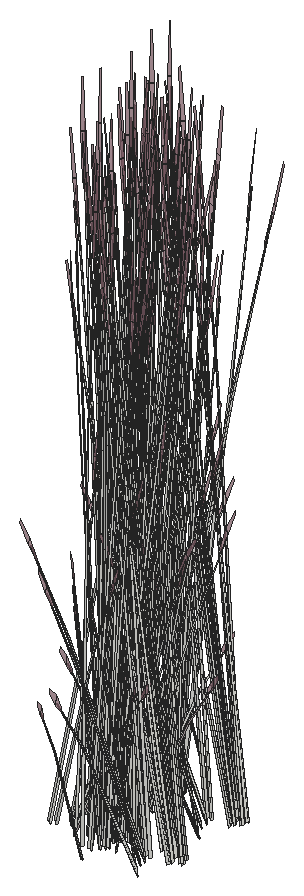
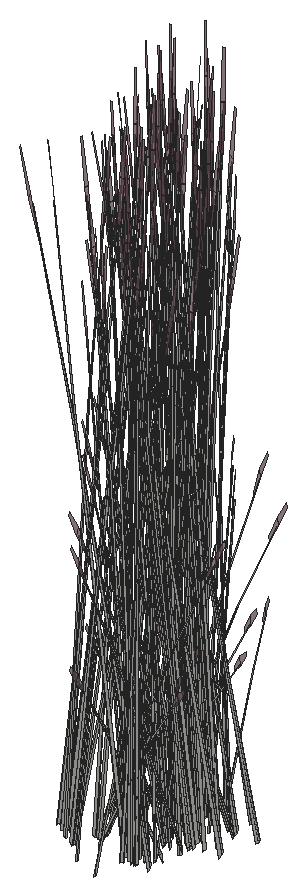
# SketchUp Ruby script. Lengths in inches.
U = 1.inch
M = Sketchup.active_model
def pt(a) = Geom::Point3d.new(a.map { |v| v * U })
def face(e, loops, mat)
  f = e.add_face(loops[0].map { |a| pt(a) })
  loops[1..].each { |l| e.add_face(l.map { |a| pt(a) }).erase! }
  f.material = f.back_material = mat if mat
  f
end
# faces: each face lists its corners as indices into pts; further lists are holes
def faces(e, pts, list, mat = nil) = list.each { |f| face(e, (f[0].is_a?(Array) ? f : [f]).map { |l| l.map { |i| pts[i] } }, mat) }
# xy, xz, yz: faces in a plane at the given z, y or x. An outline is a flat list of corners, or four numbers for a rectangle; further outlines are holes
def ring(l) = l.size == 4 ? [[l[0], l[1]], [l[2], l[1]], [l[2], l[3]], [l[0], l[3]]] : l.each_slice(2).to_a
def flat(e, list, mat, &to3) = list.each { |f| face(e, (f[0].is_a?(Array) ? f : [f]).map { |l| ring(l).map { |u, v| to3.(u, v) } }, mat) }
def xy(e, z, list, mat = nil) = flat(e, list, mat) { |x, y| [x, y, z] }
def xz(e, y, list, mat = nil) = flat(e, list, mat) { |x, z| [x, y, z] }
def yz(e, x, list, mat = nil) = flat(e, list, mat) { |y, z| [x, y, z] }
def lines(e, pts, list) = list.each { |a, b| e.add_line(pt(pts[a]), pt(pts[b])) }
# prism: a flat outline (further loops are holes) pulled along v
def prism(e, loops, v, mat = nil)
  f = face(e, loops, mat); d = Geom::Vector3d.new(v.map { |x| x * U })
  f.pushpull(f.normal.samedirection?(d) ? d.length : -d.length)
end
def box(e, o, s, mat = nil) = prism(e, [[o, [o[0] + s[0], o[1], o[2]], [o[0] + s[0], o[1] + s[1], o[2]], [o[0], o[1] + s[1], o[2]]]], [0, 0, s[2]], mat)
def at(x, y, z, deg = 0) = Geom::Transformation.translation(pt([x, y, z])) * Geom::Transformation.rotation(ORIGIN, Z_AXIS, deg.degrees)
def axes(o, x, y, z) = Geom::Transformation.new([*x, 0, *y, 0, *z, 0, *pt(o).to_a, 1])
def part(name) = M.definitions.add(name)
# library, detail: a bought-in or finely detailed component or shape, given as its bounding box
def library(name, o, s) = part(name).tap { |d| box(d.entities, o, s) }
def detail(e, o, s) = box(e.add_group.entities, o, s)
def put(e, d, t, mat = nil) = e.add_instance(d, t).tap { |i| i.material = mat if mat }
def group(e, t, mat = nil) = e.add_group.tap { |g| g.transformation = t; g.material = mat if mat }.entities
root = M.entities
M.materials.add("LightPink_Translucent").color = [144, 107, 117]
M.materials["LightPink_Translucent"].alpha = 0.75
c1 = part("blade")
p = [[2.15,0.21,22],[0,0.17,0],[0.09,0.45,0],[2.18,0.31,22],[2.29,0.31,22],[0.38,0.45,0],
  [2.48,0.24,33],[2.49,0.24,33],[2.48,0.22,33]]
faces(c1.entities,p,[[0,1,2,3],[4,5,2,3],[6,3,4,7],[8,0,3,6]])
c2 = part("seeds")
p = [[0.3,-0.1,1.38],[-0.01,-0.03,1.59],[-0.01,-0.03,0.03],[0.14,-0.07,-0.07],[0.29,-0.03,3],[0.15,0.01,3.11]]
faces(c2.entities,p,[[0,1,2,3],[1,0,4,5]],"LightPink_Translucent")
c3 = part("blade with seeds")
put(c3.entities,c1,at(0,0,0))
put(c3.entities,c2,axes([2.4,0.25,30.99],[1.5799,-0.05474,1.17369],[-0.12525,1.92788,0.29478],[-0.07173,-0.02425,1.56792]))
put(root,c3,axes([333.875,17.01,50.09],[0.63817,0.08233,0.40429],[-0.12987,0.46497,0.15865],[-0.09326,-0.0449,1.40366]))
put(root,c3,axes([332.37,20.08,50.3125],[0.47043,-0.11396,0.12794],[0.16474,0.32541,-0.36534],[0,0.07162,1.11991]))
put(root,c3,axes([329.59,16.35,49.82],[0.52523,0.06406,-0.55095],[-0.11084,0.39517,-0.1446],[0.15674,0.04788,1.21613]))
put(root,c3,axes([331.83,16.59,50],[-0.31304,-0.24986,-0.05733],[0.34284,-0.22894,-0.25992],[0.09714,-0.01612,0.85731]))
put(root,c3,axes([333.71,16.93,50.4],[-0.24498,0.3521,0.39531],[-0.50902,-0.16945,-0.19025],[0,-0.08116,1.26923]))
put(root,c3,axes([332.21,20.11,50.36],[0.56863,0.18645,-0.25709],[-0.2738,0.39352,-0.44182],[0.01787,0.09662,1.41118]))
put(root,c3,axes([331,18.77,49.79],[0.47106,0.09668,-0.27372],[-0.11861,0.34048,0.27372],[0.09497,-0.03926,1.22797]))
put(root,c3,axes([332.3125,18.36,50.29],[-0.14352,0.07909,1.26356],[-0.42983,-0.13843,-0.27174],[0.07968,-0.17216,0.54024]))
put(root,c3,axes([333.53,17.75,50.1875],[0.54257,-0.10371,0.15589],[0.13397,0.38597,0.31002],[-0.04839,-0.05624,1.41735]))
put(root,c3,axes([334.36,24.57,50.03],[-0.46965,-0.33633,-0.05417],[0.46994,-0.33653,0],[-0.0164,-0.01174,1.55135]))
put(root,c3,axes([334.23,17.82,49.94],[-0.50902,-0.17543,0],[0.24498,-0.36452,0],[0,0,1.43768]))
put(root,c3,axes([333.45,20.2,50.19],[0,-0.39075,0.43871],[0.56491,0,0],[0,0.089,1.3917]))
put(root,c3,axes([333.6875,20.56,49.78],[0,0.39075,-0.43871],[-0.56491,0,0],[0,0.089,1.3917]))
put(root,c3,axes([335.41,18.25,50.1],[0.31568,0.39156,0],[-0.52815,0.21836,-0.456],[-0.12029,0.04973,1.44655]))
put(root,c3,axes([330.89,18.61,49.78],[0.47255,-0.19538,-0.43871],[0.28245,0.35034,0],[0.10763,-0.0445,1.3917]))
put(root,c3,axes([337.74,15.88,50.29],[0.09858,0.10879,1.26356],[-0.22716,0.29571,-0.27174],[-0.23325,-0.07068,0.54024]))
put(root,c3,axes([337.74,22.16,50.29],[0.09858,0.10879,1.26356],[-0.22716,0.29571,-0.27174],[-0.23325,-0.07068,0.54024]))
put(root,c3,axes([333.7,22.125,49.32],[-0.08469,0.01408,1.55816],[-0.46834,-0.15847,-0.23804],[0.00786,-0.13218,0.26541]))
put(root,c3,axes([331.84,19.58,50.3125],[0.09741,-0.34873,0.12794],[0.4759,0.06053,-0.36534],[0.08661,0.03581,1.11991]))
put(root,c3,axes([333.42,24.18,50.09],[0.21952,0.43694,0.40429],[-0.62724,0.15194,0.15865],[0.00767,-0.08029,1.40366]))
put(root,c3,axes([333.32,24.125,49.95],[0.24498,-0.3521,-0.39531],[0.50902,0.16945,0.19025],[0,-0.08116,1.26923]))
put(root,c3,axes([335.15,17.77,50.1875],[0.14586,-0.38834,0.15589],[0.53375,0.1099,0.31002],[-0.0922,0.00189,1.41735]))
put(root,c3,axes([334.9,17.26,50.3125],[0.37303,0.23477,0.12794],[-0.31115,0.26487,-0.36534],[-0.08661,0.03581,1.11991]))
put(root,c3,axes([332.51,18.98,50.19],[-0.47255,-0.19538,0.43871],[0.28245,-0.35034,0],[0.10763,0.0445,1.3917]))
put(root,c3,axes([334.77,16.97,50.03],[-0.46965,-0.33633,-0.05417],[0.46994,-0.33653,0],[-0.0164,-0.01174,1.55135]))
put(root,c3,axes([334.89,17.09,50.4],[0.54829,-0.02412,0.39531],[0.04958,0.40041,-0.19025],[-0.09816,0.04058,1.26923]))
put(root,c3,axes([332.1,21.02,49.93],[0.53009,-0.13258,-0.16963],[0.18627,0.38191,0.00007],[0.05851,-0.01465,1.53656]))
put(root,c3,axes([335.02,18.01,50.06],[0.63212,0.12701,0.27176],[-0.15814,0.45398,-0.32244],[-0.10462,0.05682,1.45692]))
put(root,c3,axes([334.1,14.53,49.32],[-0.08469,0.01408,1.55816],[-0.46834,-0.15847,-0.23804],[0.00786,-0.13218,0.26541]))
put(root,c3,axes([337.39,16.61,49.32],[0.0128,0.06158,1.55816],[-0.25814,0.3216,-0.23804],[-0.18336,-0.01621,0.26541]))
put(root,c3,axes([337.39,22.89,49.32],[0.0128,0.06158,1.55816],[-0.25814,0.3216,-0.23804],[-0.18336,-0.01621,0.26541]))
put(root,c3,axes([335.3,17.98,50.19],[0.47255,-0.19538,0.43871],[0.28245,0.35034,0],[-0.10763,0.0445,1.3917]))
put(root,c3,axes([333.82,16.58,50.09],[0.21952,0.43694,0.40429],[-0.62724,0.15194,0.15865],[0.00767,-0.08029,1.40366]))
put(root,c3,axes([333.72,16.53,49.95],[0.24498,-0.3521,-0.39531],[0.50902,0.16945,0.19025],[0,-0.08116,1.26923]))
put(root,c3,axes([334.35,17.66,49.95],[-0.16474,-0.33688,0],[0.47043,-0.11798,0],[0,0,1.36402]))
put(root,c3,axes([333.75,18.375,49.32],[0.08172,-0.02126,1.55816],[0.49154,0.11703,-0.23804],[0.01437,0.1319,0.26541]))
put(root,c3,axes([332.11,19.88,49.95],[0.30332,0.32798,-0.39531],[-0.45944,0.23096,0.19025],[0.09816,0.04058,1.26923]))
put(root,c3,axes([334.21,24.22,49.95],[0,-0.45213,0],[0.63136,0,0],[0,0,1.58567]))
put(root,c3,axes([333.62,24.3,50.15],[0.56891,0.18939,0.21263],[-0.2738,0.39352,0.44182],[0,-0.09071,1.41855]))
put(root,c3,axes([333.44,24.04,50.4],[-0.54829,0.02412,0.39531],[-0.04958,-0.40041,-0.19025],[0.09816,-0.04058,1.26923]))
put(root,c3,axes([331.96,21.25,50.29],[0.00891,-0.12953,1.26356],[0.4258,-0.14469,-0.27174],[0.13144,0.15503,0.54024]))
put(root,c3,axes([331.45,19.41,49.82],[0.34009,-0.2937,-0.55095],[0.42248,0.26632,-0.1446],[0.13628,-0.07327,1.21613]))
put(root,c3,axes([333.18,23.35,50.1875],[-0.14586,0.38834,0.15589],[-0.53375,-0.1099,0.31002],[0.0922,-0.00189,1.41735]))
put(root,c3,axes([335.01,17,49.95],[-0.24498,0.3521,-0.39531],[-0.50902,-0.16945,0.19025],[0,0.08116,1.26923]))
put(root,c3,axes([330.9,15.89,50.29],[-0.18038,-0.01157,1.26356],[-0.18479,-0.31048,-0.27174],[0.22159,-0.08783,0.54024]))
put(root,c3,axes([337.25,18.34,49.32],[0.06773,0.03904,1.55816],[0.11484,0.36171,-0.23804],[-0.15011,0.07713,0.26541]))
put(root,c3,axes([335.98,16.78,50.1875],[-0.39671,-0.28463,0.15589],[0.39978,-0.27607,0.31002],[-0.04381,0.05813,1.41735]))
put(root,c3,axes([332.94,19.15,49.79],[0.11861,0.34048,-0.27372],[-0.47106,0.09668,0.27372],[0.09497,0.03926,1.22797]))
put(root,c3,axes([334.61,16.62,49.95],[0,-0.45213,0],[0.63136,0,0],[0,0,1.58567]))
put(root,c3,axes([333.83,20.26,50.1],[0.63136,0,0],[0,0.43672,-0.456],[0,0.09947,1.44655]))
put(root,c3,axes([332.92,22.87,50.1],[-0.31568,-0.39156,0],[0.52815,-0.21836,-0.456],[0.12029,-0.04973,1.44655]))
put(root,c3,axes([334.02,16.7,50.15],[0.56891,0.18939,0.21263],[-0.2738,0.39352,0.44182],[0,-0.09071,1.41855]))
put(root,c3,axes([334.93,16.8,50.03],[0,0.45191,-0.04981],[-0.63136,0,0],[0,0.0142,1.58489]))
put(root,c3,axes([333.84,16.4375,50.4],[-0.54829,0.02412,0.39531],[-0.04958,-0.40041,-0.19025],[0.09816,-0.04058,1.26923]))
put(root,c3,axes([331.79,19.7,50.36],[0.50979,-0.25942,-0.25709],[0.339,0.36656,-0.44182],[0.12578,0.03723,1.41118]))
put(root,c3,axes([331.23,16.92,49.75],[-0.3252,0.04689,1.25103],[-0.05176,-0.37326,0.07161],[0.22777,-0.0565,0.71188]))
put(root,c3,axes([333.02,21.88,50.36],[-0.32378,-0.01225,0.92831],[0.21383,-0.26028,0.51254],[0.12791,0.09247,0.72818]))
put(root,c3,axes([331.59,16.67,49.32],[-0.02639,-0.05932,1.55816],[0.18302,-0.34702,-0.23804],[0.18462,-0.00499,0.26541]))
put(root,c3,axes([333.58,15.75,50.1875],[-0.14586,0.38834,0.15589],[-0.53375,-0.1099,0.31002],[0.0922,-0.00189,1.41735]))
put(root,c3,axes([334.625,17.67,50.02],[0.21952,0.44891,-0.05313],[-0.62724,0.1573,0],[0.00767,0.01568,1.52132]))
put(root,c3,axes([333.91,23.93,50.09],[-0.41865,0.35461,0.40429],[-0.49737,-0.31303,0.15865],[0.10093,-0.03539,1.40366]))
put(root,c3,axes([333.32,15.27,50.1],[-0.31568,-0.39156,0],[0.52815,-0.21836,-0.456],[0.12029,-0.04973,1.44655]))
put(root,c3,axes([336.4375,17.09,49.94],[-0.63105,-0.00312,-0.04397],[0,-0.43672,0.44129],[-0.01983,0.09942,1.3992]))
put(root,c3,axes([335.2,15.77,50.1875],[-0.54257,0.10371,0.15589],[-0.13397,-0.38597,0.31002],[0.04839,0.05624,1.41735]))
put(root,c3,axes([330.5,19.47,49.41],[-0.49699,0.15644,1.13921],[-0.15819,-0.44887,0.44265],[0.30518,0.00747,1.29573]))
put(root,c3,axes([334.31,16.33,50.09],[-0.41865,0.35461,0.40429],[-0.49737,-0.31303,0.15865],[0.10093,-0.03539,1.40366]))
put(root,c3,axes([335.02,16.89,49.96],[0.35245,0.2524,0],[-0.35245,0.2524,0],[0,0,1.49564]))
put(root,c3,axes([335.54,25.9,49.32],[-0.08469,0.01408,1.55816],[-0.46834,-0.15847,-0.23804],[0.00786,-0.13218,0.26541]))
put(root,c3,axes([335.02,16.6,50.4],[0.24498,-0.3521,0.39531],[0.50902,0.16945,-0.19025],[0,0.08116,1.26923]))
put(root,c3,axes([334.81,17.82,49.95],[0.50902,0.17543,0],[-0.24498,0.36452,0],[0,0,1.54589]))
put(root,c3,axes([339.08,17.17,49.82],[-0.52523,-0.06406,-0.55095],[0.11084,-0.39517,-0.1446],[-0.15674,-0.04788,1.21613]))
put(root,c3,axes([339.08,23.44,49.82],[-0.52523,-0.06406,-0.55095],[0.11084,-0.39517,-0.1446],[-0.15674,-0.04788,1.21613]))
put(root,c3,axes([334.09,23.87,50.4],[-0.30332,-0.32798,0.39531],[0.45944,-0.23096,-0.19025],[0.09816,0.04058,1.26923]))
put(root,c3,axes([332.79,18.77,50.1],[0.31568,-0.39156,0],[0.52815,0.21836,-0.456],[0.12029,0.04973,1.44655]))
put(root,c3,axes([333.54,23.95,50.36],[-0.05884,-0.44587,-0.25709],[0.6128,-0.02696,-0.44182],[0.10791,-0.05939,1.41118]))
put(root,c3,axes([333.32,18.6,49.32],[-0.07557,-0.03078,1.55816],[-0.19412,-0.34391,-0.23804],[0.13095,-0.09333,0.26541]))
put(root,c3,axes([331.32,17.47,50.29],[-0.1216,-0.0961,1.26356],[0.15822,-0.31792,-0.27174],[0.24603,0.04307,0.54024]))
put(root,c3,axes([333.07,19.01,49.78],[0.47255,0.19538,-0.43871],[-0.28245,0.35034,0],[0.10763,0.0445,1.3917]))
put(root,c3,axes([334.85,16.51,50.1],[-0.63817,-0.08233,0.43472],[0.12987,-0.46497,0.17059],[0.09326,0.0449,1.50931]))
put(root,c3,axes([336.31,17.15,49.79],[-0.35245,0.2438,-0.27372],[-0.35245,-0.2438,0.27372],[0,0.07853,1.22797]))
put(root,c3,axes([333.05,21.79,49.32],[0.03679,-0.05641,1.55816],[0.46313,-0.16615,-0.23804],[0.14041,0.08599,0.26541]))
put(root,c3,axes([338.39,17.92,49.78],[-0.47255,-0.19538,-0.43871],[0.28245,-0.35034,0],[-0.10763,-0.0445,1.3917]))
put(root,c3,axes([338.39,24.19,49.78],[-0.47255,-0.19538,-0.43871],[0.28245,-0.35034,0],[-0.10763,-0.0445,1.3917]))
put(root,c3,axes([335.3,17.1,49.85],[0.18514,0.35777,-0.61156],[-0.53331,0.12885,-0.16051],[0.02046,0.12115,1.3499]))
put(root,c3,axes([333.46,22.96,49.79],[0.47106,0.09668,-0.27372],[-0.11861,0.34048,0.27372],[0.09497,-0.03926,1.22797]))
put(root,c3,axes([338.18,15.01,49.32],[-0.04891,0.05148,1.55816],[-0.49427,0.11098,-0.23804],[-0.1194,-0.10096,0.26541]))
put(root,c3,axes([338.18,21.28,49.32],[-0.04891,0.05148,1.55816],[-0.49427,0.11098,-0.23804],[-0.1194,-0.10096,0.26541]))
put(root,c3,axes([335.04,16.72,49.95],[0.56491,0,0],[0,0.40454,0],[0,0,1.5764]))
put(root,c3,axes([334.77,22.55,50.29],[-0.14352,0.07909,1.26356],[-0.42983,-0.13843,-0.27174],[0.07968,-0.17216,0.54024]))
put(root,c3,axes([334.49,16.27,50.4],[-0.30332,-0.32798,0.39531],[0.45944,-0.23096,-0.19025],[0.09816,0.04058,1.26923]))
put(root,c3,axes([338.68,18.16,50.1],[-0.31568,0.39156,0],[-0.52815,-0.21836,-0.456],[-0.12029,-0.04973,1.44655]))
put(root,c3,axes([338.68,24.43,50.1],[-0.31568,0.39156,0],[-0.52815,-0.21836,-0.456],[-0.12029,-0.04973,1.44655]))
put(root,c3,axes([333.94,16.35,50.36],[-0.05884,-0.44587,-0.25709],[0.6128,-0.02696,-0.44182],[0.10791,-0.05939,1.41118]))
put(root,c3,axes([335.23,16.68,50.3125],[0.47043,-0.11396,0.12794],[0.16474,0.32541,-0.36534],[0,0.07162,1.11991]))
put(root,c3,axes([332.38,19.75,49.82],[0.52523,0.06406,-0.55095],[-0.11084,0.39517,-0.1446],[0.15674,0.04788,1.21613]))
put(root,c3,axes([334.62,19.99,50],[-0.31304,-0.24986,-0.05733],[0.34284,-0.22894,-0.25992],[0.09714,-0.01612,0.85731]))
put(root,c3,axes([333.35,22.81,49.78],[0.47255,-0.19538,-0.43871],[0.28245,0.35034,0],[0.10763,-0.0445,1.3917]))
put(root,c3,axes([334.29,23.78,50.3125],[0.09741,-0.34873,0.12794],[0.4759,0.06053,-0.36534],[0.08661,0.03581,1.11991]))
put(root,c3,axes([335.07,16.71,50.36],[0.56863,0.18645,-0.25709],[-0.2738,0.39352,-0.44182],[0.01787,0.09662,1.41118]))
put(root,c3,axes([333.86,15.37,49.79],[0.47106,0.09668,-0.27372],[-0.11861,0.34048,0.27372],[0.09497,-0.03926,1.22797]))
put(root,c3,axes([338.1,18.72,50.29],[0.15933,-0.06164,1.26356],[0.39339,0.18587,-0.27174],[-0.11709,0.16083,0.54024]))
put(root,c3,axes([334.97,23.17,50.19],[-0.47255,-0.19538,0.43871],[0.28245,-0.35034,0],[0.10763,0.0445,1.3917]))
put(root,c3,axes([335.17,14.96,50.29],[-0.14352,0.07909,1.26356],[-0.42983,-0.13843,-0.27174],[0.07968,-0.17216,0.54024]))
put(root,c3,axes([337.88,15.21,49.88],[-0.14565,0.31907,-0.0344],[-0.44829,-0.09815,-0.15595],[-0.06806,-0.05219,0.51438]))
put(root,c3,axes([337.88,21.48,49.88],[-0.14565,0.31907,-0.0344],[-0.44829,-0.09815,-0.15595],[-0.06806,-0.05219,0.51438]))
put(root,c3,axes([336.31,16.8,50.19],[0,-0.39075,0.43871],[0.56491,0,0],[0,0.089,1.3917]))
put(root,c3,axes([336.55,17.16,49.78],[0,0.39075,-0.43871],[-0.56491,0,0],[0,0.089,1.3917]))
put(root,c3,axes([333.75,15.21,49.78],[0.47255,-0.19538,-0.43871],[0.28245,0.35034,0],[0.10763,-0.0445,1.3917]))
put(root,c3,axes([334.7,16.18,50.3125],[0.09741,-0.34873,0.12794],[0.4759,0.06053,-0.36534],[0.08661,0.03581,1.11991]))
put(root,c3,axes([338.55,14.81,50.29],[-0.03058,0.12783,1.26356],[-0.44698,0.10701,-0.27174],[-0.10448,-0.16522,0.54024]))
put(root,c3,axes([338.55,21.08,50.29],[-0.03058,0.12783,1.26356],[-0.44698,0.10701,-0.27174],[-0.10448,-0.16522,0.54024]))
put(root,c3,axes([339.68,17.23,50.36],[-0.50979,0.25942,-0.25709],[-0.339,-0.36656,-0.44182],[-0.12578,-0.03723,1.41118]))
put(root,c3,axes([339.68,23.5,50.36],[-0.50979,0.25942,-0.25709],[-0.339,-0.36656,-0.44182],[-0.12578,-0.03723,1.41118]))
put(root,c3,axes([335.375,15.57,50.19],[-0.47255,-0.19538,0.43871],[0.28245,-0.35034,0],[0.10763,0.0445,1.3917]))
put(root,c3,axes([337.64,16.66,50.1],[-0.63136,0,0],[0,-0.43672,-0.456],[0,-0.09947,1.44655]))
put(root,c3,axes([337.64,22.9375,50.1],[-0.63136,0,0],[0,-0.43672,-0.456],[0,-0.09947,1.44655]))
put(root,c3,axes([338.52,17.77,49.79],[-0.11861,-0.34048,-0.27372],[0.47106,-0.09668,0.27372],[-0.09497,-0.03926,1.22797]))
put(root,c3,axes([338.52,24.05,49.79],[-0.11861,-0.34048,-0.27372],[0.47106,-0.09668,0.27372],[-0.09497,-0.03926,1.22797]))
put(root,c3,axes([334.96,17.62,49.93],[0.53009,-0.13258,-0.16963],[0.18627,0.38191,0.00007],[0.05851,-0.01465,1.53656]))
put(root,c3,axes([333.91,23.61,49.82],[0.34009,-0.2937,-0.55095],[0.42248,0.26632,-0.1446],[0.13628,-0.07327,1.21613]))
put(root,c3,axes([340.02,17.51,49.82],[-0.34009,0.2937,-0.55095],[-0.42248,-0.26632,-0.1446],[-0.13628,0.07327,1.21613]))
put(root,c3,axes([338.125,16.55,50.06],[-0.46965,0.32852,0.27176],[-0.46994,-0.32506,-0.32244],[-0.0164,-0.09329,1.45692]))
put(root,c3,axes([338.125,22.82,50.06],[-0.46965,0.32852,0.27176],[-0.46994,-0.32506,-0.32244],[-0.0164,-0.09329,1.45692]))
put(root,c3,axes([334.97,16.48,49.95],[0.30332,0.32798,-0.39531],[-0.45944,0.23096,0.19025],[0.09816,0.04058,1.26923]))
put(root,c3,axes([340.25,17.35,50.18],[-0.49304,-0.31451,-0.2226],[0.41487,-0.35316,0.48713],[-0.13277,0.03679,1.48635]))
put(root,c3,axes([340.25,23.62,50.18],[-0.49304,-0.31451,-0.2226],[0.41487,-0.35316,0.48713],[-0.13277,0.03679,1.48635]))
put(root,c3,axes([339.35,17.05,49.95],[-0.30332,-0.32798,-0.39531],[0.45944,-0.23096,0.19025],[-0.09816,-0.04058,1.26923]))
put(root,c3,axes([339.35,23.32,49.95],[-0.30332,-0.32798,-0.39531],[0.45944,-0.23096,0.19025],[-0.09816,-0.04058,1.26923]))
put(root,c3,axes([334.82,17.85,50.29],[0.00891,-0.12953,1.26356],[0.4258,-0.14469,-0.27174],[0.13144,0.15503,0.54024]))
put(root,c3,axes([334.25,23.89,50.36],[0.50979,-0.25942,-0.25709],[0.339,0.36656,-0.44182],[0.12578,0.03723,1.41118]))
put(root,c3,axes([334.3125,16.01,49.82],[0.34009,-0.2937,-0.55095],[0.42248,0.26632,-0.1446],[0.13628,-0.07327,1.21613]))
put(root,c3,axes([333.69,19.29,50.29],[-0.18038,-0.01157,1.26356],[-0.18479,-0.31048,-0.27174],[0.22159,-0.08783,0.54024]))
put(root,c3,axes([340,17.28,49.95],[-0.54829,0.02412,-0.39531],[-0.04958,-0.40041,0.19025],[-0.09816,0.04058,1.26923]))
put(root,c3,axes([340,23.55,49.95],[-0.54829,0.02412,-0.39531],[-0.04958,-0.40041,0.19025],[-0.09816,0.04058,1.26923]))
put(root,c3,axes([335.8,15.75,49.79],[0.11861,0.34048,-0.27372],[-0.47106,0.09668,0.27372],[0.09497,0.03926,1.22797]))
put(root,c3,axes([336.6875,16.86,50.1],[0.63136,0,0],[0,0.43672,-0.456],[0,0.09947,1.44655]))
put(root,c3,axes([338.95,17.95,50.19],[0.47255,0.19538,0.43871],[-0.28245,0.35034,0],[-0.10763,-0.0445,1.3917]))
put(root,c3,axes([338.95,24.22,50.19],[0.47255,0.19538,0.43871],[-0.28245,0.35034,0],[-0.10763,-0.0445,1.3917]))
put(root,c3,axes([334.03,20.32,49.75],[-0.3252,0.04689,1.25103],[-0.05176,-0.37326,0.07161],[0.22777,-0.0565,0.71188]))
put(root,c3,axes([339.4,17.23,50.16],[0.13383,-0.46302,-0.20702],[0.63453,0.08071,0.45303],[-0.11087,-0.06394,1.38231]))
put(root,c3,axes([339.4,23.51,50.16],[0.13383,-0.46302,-0.20702],[0.63453,0.08071,0.45303],[-0.11087,-0.06394,1.38231]))
put(root,c3,axes([334.38,20.07,49.32],[-0.02639,-0.05932,1.55816],[0.18302,-0.34702,-0.23804],[0.18462,-0.00499,0.26541]))
put(root,c3,axes([334.65,16.3,50.36],[0.50979,-0.25942,-0.25709],[0.339,0.36656,-0.44182],[0.12578,0.03723,1.41118]))
put(root,c3,axes([332.96,23.66,49.41],[-0.49699,0.15644,1.13921],[-0.15819,-0.44887,0.44265],[0.30518,0.00747,1.29573]))
put(root,c3,axes([336.61,26.33,50.29],[-0.14352,0.07909,1.26356],[-0.42983,-0.13843,-0.27174],[0.07968,-0.17216,0.54024]))
put(root,c3,axes([335.875,18.48,50.36],[-0.32378,-0.01225,0.92831],[0.21383,-0.26028,0.51254],[0.12791,0.09247,0.72818]))
put(root,c3,axes([339.63,17.34,50.3125],[-0.09741,0.34873,0.12794],[-0.4759,-0.06053,-0.36534],[-0.08661,-0.03581,1.11991]))
put(root,c3,axes([339.63,23.62,50.3125],[-0.09741,0.34873,0.12794],[-0.4759,-0.06053,-0.36534],[-0.08661,-0.03581,1.11991]))
